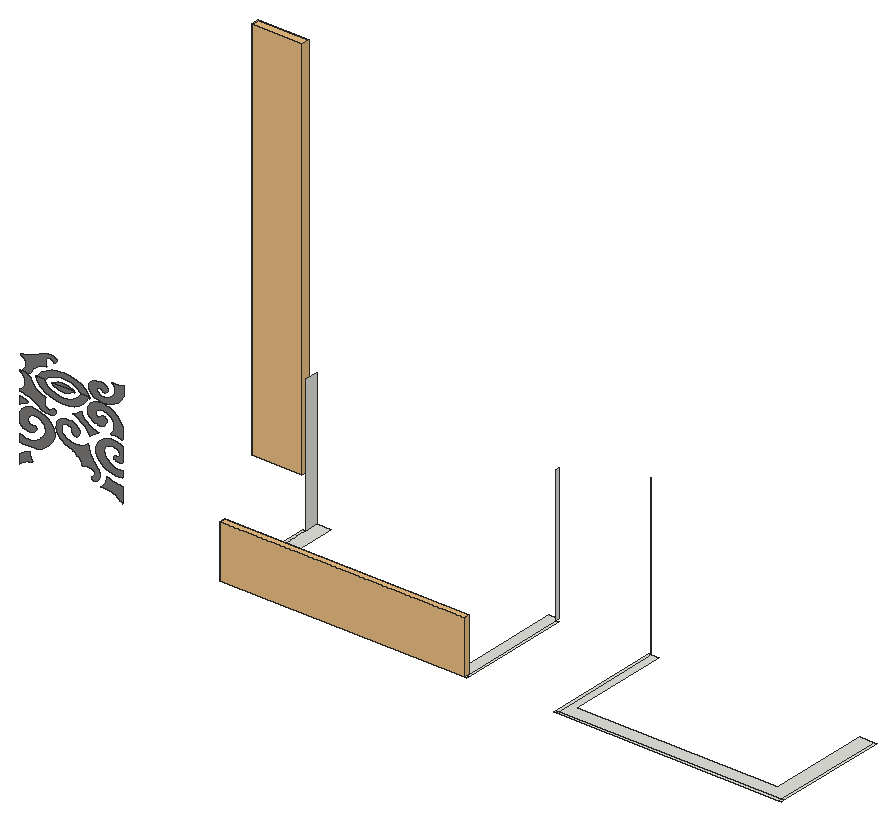
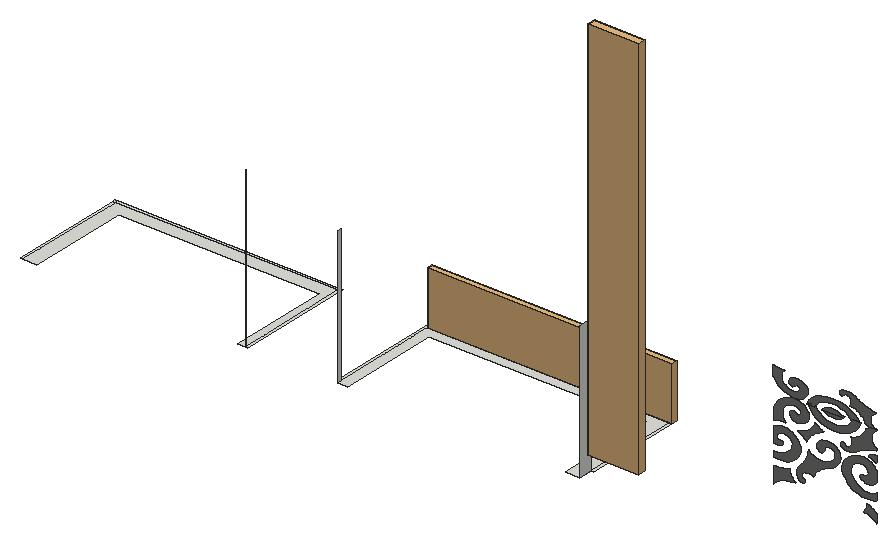
# SketchUp Ruby script. Lengths in inches.
U = 1.inch
M = Sketchup.active_model
def pt(a) = Geom::Point3d.new(a.map { |v| v * U })
def face(e, loops, mat)
  f = e.add_face(loops[0].map { |a| pt(a) })
  loops[1..].each { |l| e.add_face(l.map { |a| pt(a) }).erase! }
  f.material = f.back_material = mat if mat
  f
end
# faces: each face lists its corners as indices into pts; further lists are holes
def faces(e, pts, list, mat = nil) = list.each { |f| face(e, (f[0].is_a?(Array) ? f : [f]).map { |l| l.map { |i| pts[i] } }, mat) }
# xy, xz, yz: faces in a plane at the given z, y or x. An outline is a flat list of corners, or four numbers for a rectangle; further outlines are holes
def ring(l) = l.size == 4 ? [[l[0], l[1]], [l[2], l[1]], [l[2], l[3]], [l[0], l[3]]] : l.each_slice(2).to_a
def flat(e, list, mat, &to3) = list.each { |f| face(e, (f[0].is_a?(Array) ? f : [f]).map { |l| ring(l).map { |u, v| to3.(u, v) } }, mat) }
def xy(e, z, list, mat = nil) = flat(e, list, mat) { |x, y| [x, y, z] }
def xz(e, y, list, mat = nil) = flat(e, list, mat) { |x, z| [x, y, z] }
def yz(e, x, list, mat = nil) = flat(e, list, mat) { |y, z| [x, y, z] }
def lines(e, pts, list) = list.each { |a, b| e.add_line(pt(pts[a]), pt(pts[b])) }
# prism: a flat outline (further loops are holes) pulled along v
def prism(e, loops, v, mat = nil)
  f = face(e, loops, mat); d = Geom::Vector3d.new(v.map { |x| x * U })
  f.pushpull(f.normal.samedirection?(d) ? d.length : -d.length)
end
def box(e, o, s, mat = nil) = prism(e, [[o, [o[0] + s[0], o[1], o[2]], [o[0] + s[0], o[1] + s[1], o[2]], [o[0], o[1] + s[1], o[2]]]], [0, 0, s[2]], mat)
def at(x, y, z, deg = 0) = Geom::Transformation.translation(pt([x, y, z])) * Geom::Transformation.rotation(ORIGIN, Z_AXIS, deg.degrees)
def axes(o, x, y, z) = Geom::Transformation.new([*x, 0, *y, 0, *z, 0, *pt(o).to_a, 1])
def part(name) = M.definitions.add(name)
# library, detail: a bought-in or finely detailed component or shape, given as its bounding box
def library(name, o, s) = part(name).tap { |d| box(d.entities, o, s) }
def detail(e, o, s) = box(e.add_group.entities, o, s)
def put(e, d, t, mat = nil) = e.add_instance(d, t).tap { |i| i.material = mat if mat }
def group(e, t, mat = nil) = e.add_group.tap { |g| g.transformation = t; g.material = mat if mat }.entities
root = M.entities
M.materials.add("[0043_SaddleBrown]4").color = [124, 123, 122]
M.materials.add("[Granite Light Gray]").color = [149, 148, 144]
c1 = library("Scandinavian Door w/ Glass Wall\#2",[-41.94,78.85,0],[6.47,62.99,82.68])
c2 = library("Glass Railing",[0,0,0],[139.5,4.76,42])
xy(root,413.5,[[4301.88,557.9375,4494.32,559.875],[4494.32,557.9375,4496.26,559.875],[4564.83,557.9375,4566.77,559.875],[4566.77,557.9375,4742.06,559.875],[4742.06,557.9375,4744,559.875],
  [4301.7,559.875,4303.63,640.11],[4303.63,559.875,4494.32,559.875,4494.32,651.03,4486.46,651.03,4486.46,570.83,4314.96,570.83,4314.96,651.03,4303.63,651.03],[4494.32,559.875,4496.26,647.91],[4564.83,559.875,4566.77,651.03],[4566.77,559.875,4742.06,559.875,4742.06,651.03,4730.74,651.03,4730.74,570.83,4572.84,570.83,4572.84,651.03,4566.77,651.03],
  [4742.06,559.875,4744,651.03]])
xz(root,589.17,[[4200.24,418.4,4200.24,430.94,4199.2,430.96,4198.17,431.01,4197.13,431.09,4196.1,431.2,4195.08,431.34,4194.07,431.51,4193.07,431.7,4192.08,431.93,4191.1,432.18,4190.14,432.46,4189.1875,432.77,4188.26,433.11,4188.16,432.33,4188,431.56,4187.78,430.79,4187.52,430.03,4187.2,429.29,4186.82,428.55,4186.4,427.83,4185.93,427.13,4185.4,426.44,4184.83,425.78,4184.22,425.14,4183.56,424.52,4185.21,424.625,4186.87,424.61,4188.52,424.48,4190.14,424.22,4191.72,423.85,4193.24,423.36,4194.68,422.76,4196.03,422.0625,4197.27,421.27,4198.39,420.39,4199.39,419.43],[4119.85,418.5,4120.37,419.14,4120.96,419.74,4121.62,420.3125,4122.34,420.84,4123.11,421.32,4123.94,421.76,4124.82,422.14,4125.73,422.48,4126.68,422.75,4127.66,422.98,4128.66,423.14,4129.68,423.24,4129.26,423.73,4128.875,424.24,4128.53,424.76,4128.22,425.29,4127.95,425.83,4127.72,426.38,4127.53,426.94,4127.38,427.51,4127.27,428.08,4127.21,428.65,4127.18,429.23,4127.19,429.8,4126.5,429.54,4125.81,429.27,4125.14,428.97,4124.48,428.66,4123.84,428.33,4123.22,427.99,4122.61,427.63,4122.02,427.26,4121.45,426.87,4120.89,426.47,4120.36,426.05,4119.85,425.62],[4177.93,427.2,4178.48,427.23,4179.03,427.32,4179.55,427.46,4180.04,427.66,4180.48,427.9,4180.875,428.18,4181.21,428.51,4181.47,428.86,4181.66,429.24,4181.78,429.63,4181.82,430.04,4182.03,430.71,4182.18,431.38,4182.25,432.07,4182.26,432.76,4182.2,433.44,4182.07,434.125,4181.87,434.8,4181.6,435.46,4181.27,436.1,4180.87,436.72,4180.41,437.33,4179.89,437.9,4178.96,438.91,4178.09,439.95,4177.28,441.02,4176.54,442.11,4175.88,443.22,4175.28,444.36,4174.76,445.51,4174.3,446.68,4173.93,447.86,4173.625,449.05,4173.4,450.26,4173.25,451.46,4172.28,450.57,4171.16,449.77,4169.9,449.08,4168.54,448.52,4167.08,448.09,4165.56,447.8,4163.99,447.66,4162.42,447.66,4160.86,447.8125,4159.34,448.11,4157.88,448.54,4156.52,449.11,4155.54,449.65,4154.68,450.27,4153.93,450.97,4153.31,451.74,4152.83,452.55,4152.5,453.4,4152.32,454.28,4152.31,455.16,4152.45,456.04,4152.75,456.9,4153.19,457.72,4153.78,458.5,4154.33,458.79,4154.93,459.03,4155.57,459.19,4156.24,459.29,4156.93,459.31,4157.61,459.26,4158.27,459.13,4158.89,458.94,4159.48,458.68,4160,458.36,4160.44,457.99,4160.8125,457.57,4160.69,457.28,4160.6,456.98,4160.55,456.67,4160.53,456.37,4160.55,456.06,4160.59,455.75,4160.67,455.45,4160.79,455.16,4160.94,454.87,4161.11,454.59,4161.32,454.32,4161.56,454.0625,4161.79,453.87,4162.0625,453.7,4162.37,453.5625,4162.7,453.47,4163.05,453.41,4163.4,453.38,4163.76,453.41,4164.11,453.47,4164.44,453.5625,4164.75,453.7,4165.02,453.87,4165.25,454.0625,4165.92,454.87,4166.4,455.75,4166.65,456.67,4166.6875,457.61,4166.5,458.54,4166.09,459.4375,4165.48,460.27,4164.68,461.01,4163.71,461.64,4162.61,462.15,4161.41,462.51,4160.14,462.72,4158.72,462.91,4157.27,462.94,4155.84,462.8125,4154.45,462.53,4153.14,462.1,4151.93,461.53,4150.86,460.83,4149.94,460.03,4149.21,459.13,4148.67,458.17,4148.34,457.15,4148.23,456.12,4148.12,454.92,4148.18,453.72,4148.42,452.53,4148.82,451.37,4149.39,450.24,4150.11,449.16,4150.99,448.14,4152.01,447.19,4153.16,446.32,4154.43,445.55,4155.81,444.87,4157.27,444.3,4158.66,443.78,4159.99,443.1875,4161.27,442.53,4162.47,441.81,4163.6,441.03,4164.65,440.19,4165.62,439.31,4166.5,438.37,4167.28,437.39,4167.96,436.38,4168.55,435.33,4169.02,434.26,4169.7,434.625,4170.44,434.93,4171.23,435.15,4172.06,435.3,4172.9,435.36,4173.75,435.34,4174.59,435.24,4175.4,435.05,4176.17,434.79,4176.88,434.46,4177.53,434.06,4178.09,433.6,4178.3,433.23,4178.44,432.84,4178.53,432.45,4178.55,432.05,4178.51,431.65,4178.41,431.26,4178.25,430.875,4178.03,430.51,4177.75,430.16,4177.42,429.84,4177.04,429.55,4176.62,429.29,4176.39,429.13,4176.21,428.95,4176.08,428.75,4176,428.53,4175.99,428.3,4176.04,428.08,4176.15,427.87,4176.32,427.67,4176.53,427.51,4176.78,427.375,4177.07,427.28,4177.37,427.23],[4126.47,433.3,4128.73,433.36,4130.96,433.62,4133.14,434.07,4135.22,434.7,4137.1875,435.5,4139.01,436.47,4140.65,437.59,4142.1,438.85,4143.32,440.22,4144.99,442.26,4146.15,444.47,4146.76,446.8,4146.81,449.17,4146.28,451.51,4145.21,453.75,4143.62,455.82,4141.5625,457.67,4139.09,459.23,4136.28,460.46,4133.22,461.32,4130,461.79,4128.84,461.63,4127.71,461.4,4126.61,461.08,4125.5625,460.69,4124.57,460.24,4123.64,459.71,4122.78,459.125,4122.01,458.48,4121.32,457.79,4120.73,457.06,4120.24,456.28,4119.85,455.48,4119.85,447.4,4120.38,446.49,4121.16,445.68,4122.14,445,4123.3,444.48,4124.58,444.15,4125.93,444,4127.29,444.0625,4128.61,444.32,4129.82,444.76,4130.89,445.37,4131.76,446.13,4132.4,447,4132.49,447.21,4132.54,447.42,4132.55,447.64,4132.51,447.86,4132.42,448.07,4132.3,448.27,4132.13,448.46,4131.93,448.62,4131.7,448.76,4131.44,448.88,4131.16,448.97,4130.87,449.02,4130.14,448.93,4129.4,448.94,4128.68,449.05,4128,449.25,4127.38,449.54,4126.84,449.9,4126.41,450.33,4126.09,450.81,4125.9,451.32,4125.85,451.85,4125.93,452.38,4126.15,452.89,4126.33,453.55,4126.65,454.18,4127.11,454.77,4127.69,455.29,4128.38,455.75,4129.16,456.12,4130.01,456.4,4130.91,456.57,4131.84,456.65,4132.77,456.62,4133.68,456.48,4134.55,456.24,4135.91,455.45,4137.1,454.53,4138.09,453.51,4138.88,452.39,4139.4375,451.2,4139.75,449.96,4139.83,448.71,4139.65,447.46,4139.24,446.24,4138.58,445.08,4137.71,443.99,4136.63,443.01,4136.19,442.35,4135.68,441.73,4135.1,441.14,4134.45,440.59,4133.74,440.07,4132.97,439.6,4132.15,439.18,4131.29,438.8125,4130.39,438.49,4129.45,438.23,4128.48,438.03,4127.5,437.88,4126.8,437.82,4126.09,437.8,4125.39,437.83,4124.6875,437.89,4124,438,4123.32,438.16,4122.67,438.35,4122.04,438.58,4121.4375,438.85,4120.87,439.15,4120.34,439.48,4119.85,439.85,4119.85,434.28,4122,433.76,4124.21,433.44],[4197.64,436.71,4200.24,436.96,4200.24,441.66,4198.01,441.61,4195.8,441.84,4193.68,442.34,4191.71,443.09,4189.96,444.09,4188.47,445.28,4187.29,446.65,4186.46,448.14,4186,449.72,4185.92,451.32,4186.24,452.92,4186.9375,454.45,4187.73,455.1,4188.68,455.63,4189.76,456.03,4190.92,456.27,4192.12,456.35,4193.32,456.27,4194.48,456.02,4195.55,455.625,4196.5,455.09,4197.29,454.43,4197.9,453.68,4198.3,452.86,4198.375,452.53,4198.37,452.1875,4198.28,451.86,4198.12,451.54,4197.88,451.25,4197.58,450.99,4197.22,450.77,4196.8125,450.61,4196.375,450.49,4195.91,450.43,4195.45,450.42,4194.98,450.48,4194.74,450.4,4194.51,450.31,4194.3,450.19,4194.11,450.06,4193.93,449.92,4193.78,449.77,4193.65,449.6,4193.55,449.42,4193.47,449.24,4193.42,449.06,4193.4,448.87,4193.41,448.68,4193.78,448.29,4194.22,447.9375,4194.71,447.63,4195.26,447.38,4195.85,447.18,4196.48,447.04,4197.12,446.96,4197.77,446.9375,4198.42,446.98,4199.05,447.09,4199.67,447.25,4200.24,447.47,4200.24,459.11,4199.18,459.72,4198.02,460.23,4196.79,460.64,4195.49,460.9375,4194.16,461.12,4192.8,461.18,4191.44,461.12,4190.11,460.9375,4188.8125,460.64,4187.58,460.23,4186.42,459.72,4185.36,459.11,4184.47,458.48,4183.63,457.82,4182.86,457.11,4182.16,456.375,4181.53,455.6,4180.97,454.8,4180.48,453.97,4180.08,453.125,4179.75,452.26,4179.51,451.38,4179.34,450.49,4179.26,449.6,4179.38,447.71,4179.89,445.86,4180.78,444.08,4182.03,442.42,4183.61,440.92,4185.49,439.6,4187.62,438.5,4189.95,437.65,4192.44,437.06,4195.03,436.74],
  [4174.35,457.23,4174.9,457.6875,4175.46,458.14,4176.03,458.59,4176.61,459.03,4177.2,459.46,4177.8,459.89,4178.42,460.31,4179.04,460.72,4179.66,461.12,4180.3,461.52,4180.95,461.91,4181.61,462.29,4179.94,462.61,4178.33,463.04,4176.79,463.58,4175.33,464.23,4173.96,464.99,4172.71,465.83,4171.57,466.76,4170.57,467.77,4169.71,468.84,4168.99,469.96,4168.44,471.14,4168.05,472.34,4167.56,471.93,4167.0625,471.54,4166.54,471.16,4166,470.79,4165.4375,470.43,4164.86,470.09,4164.26,469.77,4163.65,469.47,4163.02,469.18,4162.38,468.9,4161.73,468.65,4161.0625,468.41,4162.625,467.83,4164.13,467.18,4165.5625,466.45,4166.92,465.65,4168.2,464.79,4169.39,463.86,4170.48,462.87,4171.47,461.83,4172.36,460.74,4173.14,459.6,4173.8,458.43],[4119.85,460.92,4120.27,461.25,4120.7,461.57,4121.16,461.88,4121.63,462.17,4122.125,462.45,4122.63,462.71,4123.15,462.95,4123.69,463.18,4124.24,463.39,4124.81,463.58,4125.38,463.75,4125.97,463.91,4125.59,464.24,4125.17,464.55,4124.73,464.84,4124.27,465.11,4123.77,465.35,4123.26,465.56,4122.72,465.76,4122.17,465.92,4121.61,466.05,4121.03,466.16,4120.44,466.24,4119.85,466.28],[4141.9,461.65,4142.82,461.6875,4143.73,461.8,4144.62,461.98,4145.48,462.23,4145.78,462.34,4146.07,462.47,4146.35,462.62,4146.6,462.79,4146.84,462.96,4147.05,463.16,4147.24,463.36,4147.41,463.58,4147.55,463.8,4147.67,464.03,4147.76,464.27,4147.82,464.52,4147.84,464.75,4147.83,464.99,4147.78,465.23,4147.69,465.46,4147.57,465.6875,4147.41,465.9,4147.22,466.1,4147,466.28,4146.75,466.4375,4146.48,466.58,4146.1875,466.69,4145.88,466.78,4145.6875,466.54,4145.48,466.29,4145.27,466.06,4145.04,465.83,4144.8,465.6,4144.55,465.38,4144.29,465.17,4144.02,464.96,4143.74,464.77,4143.45,464.57,4143.16,464.39,4142.85,464.21,4142.42,464.28,4142.01,464.375,4141.61,464.5,4141.23,464.65,4140.875,464.83,4140.54,465.03,4140.24,465.26,4139.97,465.5,4139.73,465.77,4139.53,466.04,4139.37,466.33,4139.24,466.63,4139.1,467.11,4138.99,467.58,4138.92,468.0625,4138.87,468.55,4138.86,469.03,4138.88,469.51,4138.9375,469.99,4139.02,470.47,4139.14,470.95,4139.29,471.42,4139.48,471.88,4139.69,472.34,4138.22,472.75,4136.8125,473.24,4135.46,473.83,4134.2,474.5,4133.01,475.24,4131.93,476.0625,4130.95,476.95,4130.09,477.9,4129.34,478.89,4128.72,479.94,4128.24,481.01,4127.88,482.12,4127.5,482.3,4127.13,482.48,4126.41,482.88,4126.0625,483.09,4125.72,483.31,4125.39,483.53,4125.07,483.77,4124.76,484.01,4124.47,484.25,4124.18,484.5,4123.9,484.8,4119.85,484.8,4119.85,483.92,4120.9375,483.03,4121.85,482.05,4122.58,480.99,4123.11,479.87,4123.4375,478.71,4123.54,477.53,4123.4375,476.35,4123.11,475.1875,4122.58,474.07,4121.85,473.01,4120.9375,472.02,4119.85,471.14,4119.85,469.95,4121.32,469.73,4122.78,469.45,4124.21,469.11,4125.61,468.72,4126.98,468.27,4128.32,467.77,4129.61,467.21,4130.86,466.61,4132.0625,465.96,4133.21,465.26,4134.31,464.51,4135.34,463.73,4136,463.26,4136.71,462.84,4137.49,462.48,4138.3125,462.18,4139.18,461.94,4140.07,461.77,4140.98,461.68],[4200.24,463.51,4200.24,472.52,4199.83,473.85,4199.23,475.15,4198.47,476.4,4197.55,477.6,4196.46,478.72,4195.24,479.76,4193.88,480.71,4192.4,481.57,4190.81,482.3125,4189.13,482.95,4187.375,483.46,4185.56,483.85,4183.89,483.91,4182.23,483.79,4180.61,483.49,4179.07,483.03,4177.65,482.4,4176.36,481.63,4175.26,480.73,4174.34,479.72,4173.65,478.625,4173.19,477.47,4172.97,476.28,4173,475.07,4172.95,474.3125,4173.04,473.55,4173.24,472.81,4173.58,472.09,4174.03,471.4,4174.59,470.76,4175.26,470.17,4176.03,469.64,4176.87,469.1875,4177.79,468.81,4178.76,468.51,4179.78,468.31,4180.45,468.02,4181.19,467.82,4181.96,467.71,4182.75,467.7,4183.53,467.78,4184.27,467.96,4184.97,468.22,4185.59,468.57,4186.12,468.99,4186.54,469.47,4186.85,469.99,4187.02,470.54,4187.42,470.95,4187.72,471.4,4187.9,471.88,4187.97,472.38,4187.91,472.88,4187.74,473.36,4187.46,473.81,4187.07,474.23,4186.59,474.59,4186.03,474.88,4185.41,475.1,4184.75,475.24,4184.51,474.99,4184.27,474.75,4183.75,474.29,4183.47,474.07,4183.1875,473.85,4182.89,473.64,4182.59,473.44,4182.27,473.25,4181.95,473.0625,4181.62,472.88,4181.28,472.71,4180.91,472.88,4180.56,473.08,4180.25,473.31,4179.97,473.55,4179.73,473.82,4179.53,474.1,4179.38,474.4,4179.27,474.71,4179.21,475.02,4179.19,475.34,4179.22,475.66,4179.31,475.97,4179.59,476.6,4180.02,477.18,4180.5625,477.71,4181.22,478.17,4181.98,478.54,4182.8,478.83,4183.68,479.01,4184.59,479.09,4185.51,479.06,4186.41,478.93,4187.26,478.7,4188.05,478.36,4189.47,477.55,4190.72,476.6,4191.78,475.54,4192.64,474.39,4193.26,473.16,4193.66,471.88,4193.81,470.58,4193.71,469.28,4193.375,467.99,4192.8,466.75,4192,465.58,4190.98,464.5,4191.76,464.63,4192.55,464.73,4193.35,464.78,4194.16,464.8,4194.96,464.77,4195.76,464.71,4196.55,464.6,4197.32,464.46,4198.08,464.28,4198.83,464.06,4199.55,463.8],[4153.08,472.34,4157.91,472.75,4162.47,473.95,4166.52,475.88,4169.85,478.43,4172.29,481.46,4173.6875,484.8,4167.53,484.8,4166.35,482.62,4164.54,480.66,4162.19,479.03,4159.41,477.8,4156.32,477.04,4153.08,476.77,4149.83,477.02,4146.74,477.76,4143.9375,478.97,4141.57,480.59,4139.73,482.53,4138.53,484.8,4132.37,484.8,4133.8,481.37,4136.26,478.35,4139.61,475.82,4143.6875,473.91,4148.26,472.73],
  [4153.4,480.9,4155.16,481.02,4156.86,481.375,4158.4375,481.95,4159.83,482.74,4161,483.7,4161.9,484.8,4144.9,484.8,4145.8,483.7,4146.96,482.74,4148.36,481.95,4149.9375,481.375,4151.64,481.02],[4120.56,483.9,4120.56,484.65,4121.64,485.41,4122.5625,486.24,4123.29,487.15,4123.82,488.1,4124.14,489.09,4124.25,490.1,4124.14,491.1,4123.82,492.09,4123.29,493.05,4122.5625,493.95,4121.64,494.79,4120.56,495.54,4120.56,496.56,4122.03,496.75,4123.48,496.98,4124.92,497.27,4126.32,497.61,4127.6875,497.99,4129.02,498.41,4130.32,498.89,4131.57,499.4,4132.77,499.96,4133.92,500.55,4135.01,501.1875,4136.05,501.86,4136.7,502.26,4137.42,502.61,4138.2,502.92,4139.02,503.18,4139.88,503.375,4140.78,503.52,4141.6875,503.6,4142.61,503.63,4143.53,503.59,4144.44,503.5,4145.33,503.34,4146.18,503.13,4146.49,503.04,4146.78,502.92,4147.05,502.8,4147.31,502.66,4147.54,502.51,4147.76,502.34,4147.95,502.17,4148.12,501.98,4148.26,501.79,4148.375,501.59,4148.46,501.39,4148.52,501.18,4148.55,500.98,4148.54,500.78,4148.49,500.57,4148.4,500.375,4148.28,500.1875,4148.12,500.01,4147.93,499.84,4147.71,499.68,4147.46,499.55,4147.1875,499.43,4146.9,499.33,4146.59,499.25,4146.19,499.67,4145.75,500.07,4145.51,500.26,4145.26,500.44,4145,500.625,4144.73,500.8,4144.45,500.97,4144.16,501.13,4143.86,501.29,4143.56,501.44,4143.13,501.38,4142.72,501.3,4142.32,501.2,4141.94,501.07,4141.58,500.91,4141.25,500.74,4140.95,500.55,4140.68,500.34,4140.4375,500.12,4140.24,499.88,4140.07,499.64,4139.95,499.38,4139.81,498.98,4139.7,498.57,4139.625,498.16,4139.58,497.75,4139.57,497.34,4139.59,496.93,4139.64,496.52,4139.73,496.11,4139.85,495.7,4140,495.3,4140.18,494.91,4140.4,494.52,4138.93,494.17,4137.52,493.75,4136.17,493.25,4134.9,492.68,4133.72,492.05,4132.64,491.35,4131.66,490.59,4130.79,489.78,4130.05,488.93,4129.43,488.05,4128.94,487.13,4128.59,486.1875,4128.21,486.04,4127.84,485.88,4127.47,485.71,4127.12,485.54,4126.77,485.36,4126.43,485.17,4126.1,484.98,4125.78,484.78,4125.47,484.58,4125.17,484.37,4124.88,484.16,4124.6,483.9],[4133.08,483.9,4134.51,486.82,4136.97,489.4,4140.32,491.55,4144.39,493.18,4148.96,494.1875,4153.79,494.52,4158.61,494.17,4163.17,493.14,4167.23,491.5,4170.5625,489.33,4172.99,486.75,4174.4,483.9,4168.24,483.9,4167.06,485.76,4165.25,487.43,4162.9,488.82,4160.11,489.86,4157.03,490.51,4153.79,490.74,4150.54,490.53,4147.45,489.9,4144.65,488.87,4142.27,487.49,4140.44,485.83,4139.23,483.9],[4145.61,483.9,4146.5,484.84,4147.67,485.66,4149.07,486.33,4150.64,486.82,4152.34,487.125,4154.11,487.23,4155.87,487.125,4157.57,486.82,4159.15,486.33,4160.54,485.66,4161.71,484.84,4162.6,483.9],[4184.6,484.66,4182.9375,484.76,4181.32,485.02,4179.78,485.41,4178.35,485.95,4177.07,486.6,4175.96,487.37,4175.05,488.23,4174.36,489.16,4173.9,490.15,4173.68,491.16,4173.71,492.1875,4173.66,492.84,4173.74,493.48,4173.95,494.12,4174.28,494.73,4174.74,495.32,4175.3,495.87,4175.97,496.37,4176.73,496.82,4177.58,497.21,4178.5,497.53,4179.47,497.78,4180.49,497.95,4181.16,498.2,4181.9,498.37,4182.67,498.46,4183.46,498.48,4184.23,498.4,4184.98,498.25,4185.67,498.02,4186.3,497.73,4186.83,497.37,4187.25,496.96,4187.55,496.52,4187.73,496.05,4188.13,495.7,4188.43,495.32,4188.61,494.91,4188.68,494.48,4188.62,494.0625,4188.45,493.65,4188.17,493.26,4187.78,492.91,4187.3,492.6,4186.74,492.35,4186.12,492.17,4185.45,492.05,4185.22,492.26,4184.98,492.46,4184.46,492.86,4184.18,493.05,4183.6,493.41,4183.29,493.58,4182.98,493.74,4182.66,493.9,4182.32,494.05,4181.99,494.2,4181.61,494.05,4181.27,493.89,4180.95,493.7,4180.68,493.49,4180.4375,493.26,4180.24,493.02,4180.08,492.76,4179.98,492.5,4179.91,492.23,4179.9,491.96,4179.93,491.69,4180.01,491.43,4180.3,490.89,4180.72,490.39,4181.27,489.94,4181.93,489.55,4182.68,489.23,4183.51,488.99,4184.39,488.83,4185.3,488.77,4186.22,488.79,4187.11,488.9,4187.97,489.1,4188.76,489.39,4190.18,490.08,4191.43,490.89,4192.49,491.79,4193.34,492.77,4193.97,493.82,4194.37,494.91,4194.52,496.02,4194.42,497.13,4194.08,498.22,4193.51,499.28,4192.7,500.28,4191.69,501.2,4192.47,501.09,4193.26,501.01,4194.0625,500.96,4194.86,500.95,4195.67,500.97,4196.46,501.02,4197.25,501.11,4198.03,501.23,4198.79,501.39,4199.53,501.57,4200.25,501.79,4200.95,502.04,4200.95,494.37,4200.53,493.23,4199.94,492.125,4199.18,491.06,4198.25,490.04,4197.17,489.08,4195.95,488.2,4194.59,487.38,4193.11,486.66,4191.52,486.02,4189.84,485.48,4188.08,485.04,4186.26,484.71]],"[0043_SaddleBrown]4")
xz(root,651.03,[[4566.56,413.5,4566.77,538.1875]])
yz(root,4303.63,[[640.11,413.5,651.03,520.4375]])
yz(root,4494.32,[[647.91,413.5,651.03,520.4375]])
p = [[4119.85,589.17,469.95],[4119.85,589.17,466.28]]
lines(root,p,[[0,1]])
put(root,c1,axes([4198.12,621.1,440.32],[0,-1,0],[0.63229,0,0],[0,0,3.672]))
put(root,c2,axes([4301.88,557.9375,413.5],[1.37946,0,0],[0,1,0],[0,0,1]),"[Granite Light Gray]")
